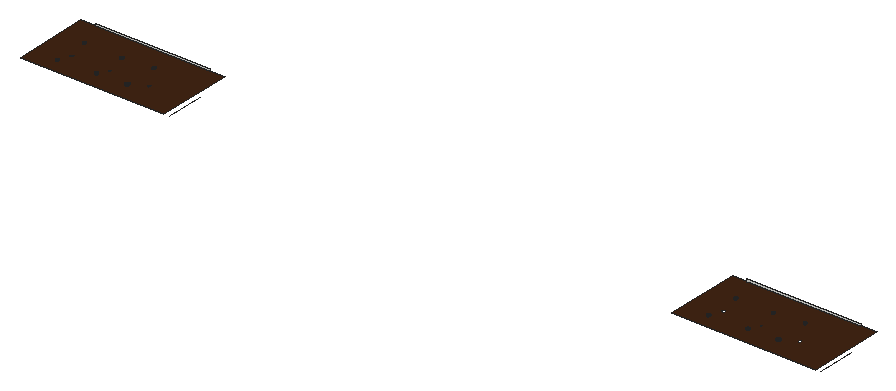
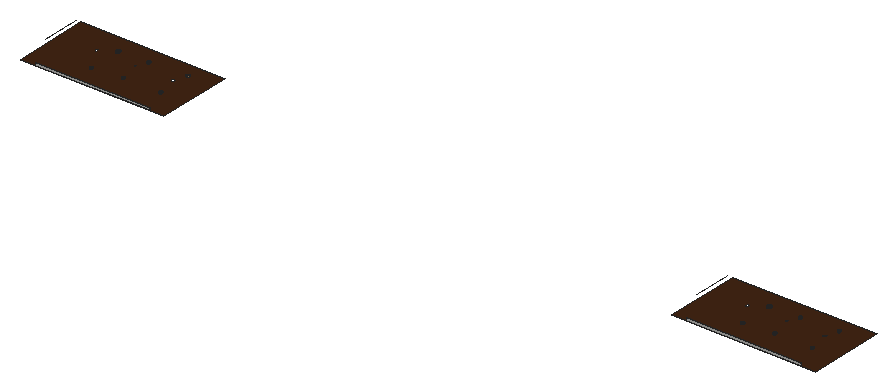
# SketchUp Ruby script. Lengths in inches.
U = 1.inch
M = Sketchup.active_model
def pt(a) = Geom::Point3d.new(a.map { |v| v * U })
def face(e, loops, mat)
  f = e.add_face(loops[0].map { |a| pt(a) })
  loops[1..].each { |l| e.add_face(l.map { |a| pt(a) }).erase! }
  f.material = f.back_material = mat if mat
  f
end
# faces: each face lists its corners as indices into pts; further lists are holes
def faces(e, pts, list, mat = nil) = list.each { |f| face(e, (f[0].is_a?(Array) ? f : [f]).map { |l| l.map { |i| pts[i] } }, mat) }
# xy, xz, yz: faces in a plane at the given z, y or x. An outline is a flat list of corners, or four numbers for a rectangle; further outlines are holes
def ring(l) = l.size == 4 ? [[l[0], l[1]], [l[2], l[1]], [l[2], l[3]], [l[0], l[3]]] : l.each_slice(2).to_a
def flat(e, list, mat, &to3) = list.each { |f| face(e, (f[0].is_a?(Array) ? f : [f]).map { |l| ring(l).map { |u, v| to3.(u, v) } }, mat) }
def xy(e, z, list, mat = nil) = flat(e, list, mat) { |x, y| [x, y, z] }
def xz(e, y, list, mat = nil) = flat(e, list, mat) { |x, z| [x, y, z] }
def yz(e, x, list, mat = nil) = flat(e, list, mat) { |y, z| [x, y, z] }
def lines(e, pts, list) = list.each { |a, b| e.add_line(pt(pts[a]), pt(pts[b])) }
# prism: a flat outline (further loops are holes) pulled along v
def prism(e, loops, v, mat = nil)
  f = face(e, loops, mat); d = Geom::Vector3d.new(v.map { |x| x * U })
  f.pushpull(f.normal.samedirection?(d) ? d.length : -d.length)
end
def box(e, o, s, mat = nil) = prism(e, [[o, [o[0] + s[0], o[1], o[2]], [o[0] + s[0], o[1] + s[1], o[2]], [o[0], o[1] + s[1], o[2]]]], [0, 0, s[2]], mat)
def at(x, y, z, deg = 0) = Geom::Transformation.translation(pt([x, y, z])) * Geom::Transformation.rotation(ORIGIN, Z_AXIS, deg.degrees)
def axes(o, x, y, z) = Geom::Transformation.new([*x, 0, *y, 0, *z, 0, *pt(o).to_a, 1])
def part(name) = M.definitions.add(name)
# library, detail: a bought-in or finely detailed component or shape, given as its bounding box
def library(name, o, s) = part(name).tap { |d| box(d.entities, o, s) }
def detail(e, o, s) = box(e.add_group.entities, o, s)
def put(e, d, t, mat = nil) = e.add_instance(d, t).tap { |i| i.material = mat if mat }
def group(e, t, mat = nil) = e.add_group.tap { |g| g.transformation = t; g.material = mat if mat }.entities
root = M.entities
M.materials.add("[Field Square Tile]").color = [211, 167, 108]
M.materials.add("[Wood Veneer 01]").color = [66, 38, 20]
xy(root,251.5,[[[1990.46,2294.125,2184.6,2396.68],[2030.6,2327.89,2031.39,2328,2032.13,2328.3,2032.76,2328.79,2033.25,2329.43,2033.56,2330.16,2033.66,2330.96,2033.56,2331.75,2033.25,2332.49,2032.76,2333.12,2032.13,2333.61,2031.39,2333.91,2030.6,2334.02,2029.81,2333.91,2029.07,2333.61,2028.43,2333.12,2027.95,2332.49,2027.64,2331.75,2027.54,2330.96,2027.64,2330.16,2027.95,2329.43,2028.43,2328.79,2029.07,2328.3,2029.81,2328],[2134.54,2328.21,2135.25,2328.3,2135.92,2328.57,2136.49,2329.01,2136.92,2329.58,2137.2,2330.24,2137.29,2330.96,2137.2,2331.67,2136.92,2332.33,2136.49,2332.9,2135.92,2333.34,2135.25,2333.61,2134.54,2333.71,2133.83,2333.61,2133.17,2333.34,2132.6,2332.9,2132.16,2332.33,2131.89,2331.67,2131.79,2330.96,2131.89,2330.24,2132.16,2329.58,2132.6,2329.01,2133.17,2328.57,2133.83,2328.3],[2081.97,2328.39,2082.63,2328.48,2083.25,2328.74,2083.78,2329.14,2084.19,2329.68,2084.45,2330.29,2084.53,2330.96,2084.45,2331.62,2084.19,2332.24,2083.78,2332.77,2083.25,2333.18,2082.63,2333.43,2081.97,2333.52,2081.31,2333.43,2080.69,2333.18,2080.16,2332.77,2079.75,2332.24,2079.5,2331.62,2079.41,2330.96,2079.5,2330.29,2079.75,2329.68,2080.16,2329.14,2080.69,2328.74,2081.31,2328.48],[2114.7,2316.65,2115.33,2316.73,2115.92,2316.97,2116.42,2317.36,2116.81,2317.87,2117.05,2318.45,2117.13,2319.08,2117.05,2319.72,2116.81,2320.3,2116.42,2320.81,2115.92,2321.2,2115.33,2321.4375,2114.7,2321.52,2114.07,2321.4375,2113.48,2321.2,2112.97,2320.81,2112.59,2320.3,2112.34,2319.72,2112.26,2319.08,2112.34,2318.45,2112.59,2317.87,2112.97,2317.36,2113.48,2316.97,2114.07,2316.73],[2074.74,2358.2,2075.22,2358.27,2075.67,2358.46,2076.0625,2358.75,2076.36,2359.14,2076.55,2359.59,2076.61,2360.08,2076.55,2360.56,2076.36,2361.02,2076.0625,2361.41,2075.67,2361.7,2075.22,2361.89,2074.74,2361.95,2074.25,2361.89,2073.8,2361.7,2073.41,2361.41,2073.11,2361.02,2072.92,2360.56,2072.86,2360.08,2072.92,2359.59,2073.11,2359.14,2073.41,2358.75,2073.8,2358.46,2074.25,2358.27],[2074.74,2315.39,2075.22,2315.46,2075.67,2315.64,2076.0625,2315.94,2076.36,2316.33,2076.55,2316.78,2076.61,2317.27,2076.55,2317.75,2076.36,2318.2,2076.0625,2318.59,2075.67,2318.89,2075.22,2319.08,2074.74,2319.14,2074.25,2319.08,2073.8,2318.89,2073.41,2318.59,2073.11,2318.2,2072.92,2317.75,2072.86,2317.27,2072.92,2316.78,2073.11,2316.33,2073.41,2315.94,2073.8,2315.64,2074.25,2315.46],[2024.3,2358.2,2024.78,2358.27,2025.24,2358.46,2025.625,2358.75,2025.92,2359.14,2026.11,2359.59,2026.17,2360.08,2026.11,2360.56,2025.92,2361.02,2025.625,2361.41,2025.24,2361.7,2024.78,2361.89,2024.3,2361.95,2023.8125,2361.89,2023.36,2361.7,2022.97,2361.41,2022.67,2361.02,2022.49,2360.56,2022.42,2360.08,2022.49,2359.59,2022.67,2359.14,2022.97,2358.75,2023.36,2358.46,2023.8125,2358.27],[2024.3,2312.27,2024.78,2312.33,2025.24,2312.52,2025.625,2312.82,2025.92,2313.2,2026.11,2313.66,2026.17,2314.14,2026.11,2314.63,2025.92,2315.08,2025.625,2315.47,2025.24,2315.77,2024.78,2315.95,2024.3,2316.02,2023.8125,2315.95,2023.36,2315.77,2022.97,2315.47,2022.67,2315.08,2022.49,2314.63,2022.42,2314.14,2022.49,2313.66,2022.67,2313.2,2022.97,2312.82,2023.36,2312.52,2023.8125,2312.33],[2114.7,2362.38,2115.13,2362.4375,2115.54,2362.6,2115.89,2362.87,2116.16,2363.22,2116.33,2363.63,2116.38,2364.07,2116.33,2364.5,2116.16,2364.91,2115.89,2365.26,2115.54,2365.53,2115.13,2365.7,2114.7,2365.75,2114.26,2365.7,2113.85,2365.53,2113.5,2365.26,2113.24,2364.91,2113.07,2364.5,2113.01,2364.07,2113.07,2363.63,2113.24,2363.22,2113.5,2362.87,2113.85,2362.6,2114.26,2362.4375]],[[2869.21,2294.125,3063.35,2396.68],[2909.35,2327.89,2910.14,2328,2910.88,2328.3,2911.51,2328.79,2912,2329.43,2912.31,2330.16,2912.41,2330.96,2912.31,2331.75,2912,2332.49,2911.51,2333.12,2910.88,2333.61,2910.14,2333.91,2909.35,2334.02,2908.56,2333.91,2907.82,2333.61,2907.18,2333.12,2906.7,2332.49,2906.39,2331.75,2906.29,2330.96,2906.39,2330.16,2906.7,2329.43,2907.18,2328.79,2907.82,2328.3,2908.56,2328],[3013.29,2328.21,3014,2328.3,3014.67,2328.57,3015.24,2329.01,3015.67,2329.58,3015.95,2330.24,3016.04,2330.96,3015.95,2331.67,3015.67,2332.33,3015.24,2332.9,3014.67,2333.34,3014,2333.61,3013.29,2333.71,3012.58,2333.61,3011.92,2333.34,3011.35,2332.9,3010.91,2332.33,3010.64,2331.67,3010.54,2330.96,3010.64,2330.24,3010.91,2329.58,3011.35,2329.01,3011.92,2328.57,3012.58,2328.3],[2960.72,2328.39,2961.38,2328.48,2962,2328.74,2962.53,2329.14,2962.94,2329.68,2963.2,2330.29,2963.28,2330.96,2963.2,2331.62,2962.94,2332.24,2962.53,2332.77,2962,2333.18,2961.38,2333.43,2960.72,2333.52,2960.06,2333.43,2959.44,2333.18,2958.91,2332.77,2958.5,2332.24,2958.25,2331.62,2958.16,2330.96,2958.25,2330.29,2958.5,2329.68,2958.91,2329.14,2959.44,2328.74,2960.06,2328.48],[2993.45,2316.65,2994.08,2316.73,2994.67,2316.97,2995.17,2317.36,2995.56,2317.87,2995.8,2318.45,2995.88,2319.08,2995.8,2319.72,2995.56,2320.3,2995.17,2320.81,2994.67,2321.2,2994.08,2321.4375,2993.45,2321.52,2992.82,2321.4375,2992.23,2321.2,2991.72,2320.81,2991.34,2320.3,2991.09,2319.72,2991.01,2319.08,2991.09,2318.45,2991.34,2317.87,2991.72,2317.36,2992.23,2316.97,2992.82,2316.73],[2903.05,2358.2,2903.53,2358.27,2903.99,2358.46,2904.375,2358.75,2904.67,2359.14,2904.86,2359.59,2904.92,2360.08,2904.86,2360.56,2904.67,2361.02,2904.375,2361.41,2903.99,2361.7,2903.53,2361.89,2903.05,2361.95,2902.5625,2361.89,2902.11,2361.7,2901.72,2361.41,2901.42,2361.02,2901.24,2360.56,2901.17,2360.08,2901.24,2359.59,2901.42,2359.14,2901.72,2358.75,2902.11,2358.46,2902.5625,2358.27],[2953.49,2358.2,2953.97,2358.27,2954.42,2358.46,2954.8125,2358.75,2955.11,2359.14,2955.3,2359.59,2955.36,2360.08,2955.3,2360.56,2955.11,2361.02,2954.8125,2361.41,2954.42,2361.7,2953.97,2361.89,2953.49,2361.95,2953,2361.89,2952.55,2361.7,2952.16,2361.41,2951.86,2361.02,2951.67,2360.56,2951.61,2360.08,2951.67,2359.59,2951.86,2359.14,2952.16,2358.75,2952.55,2358.46,2953,2358.27],[2953.49,2315.39,2953.97,2315.46,2954.42,2315.64,2954.8125,2315.94,2955.11,2316.33,2955.3,2316.78,2955.36,2317.27,2955.3,2317.75,2955.11,2318.2,2954.8125,2318.59,2954.42,2318.89,2953.97,2319.08,2953.49,2319.14,2953,2319.08,2952.55,2318.89,2952.16,2318.59,2951.86,2318.2,2951.67,2317.75,2951.61,2317.27,2951.67,2316.78,2951.86,2316.33,2952.16,2315.94,2952.55,2315.64,2953,2315.46],[2903.05,2312.27,2903.53,2312.33,2903.99,2312.52,2904.375,2312.82,2904.67,2313.2,2904.86,2313.66,2904.92,2314.14,2904.86,2314.63,2904.67,2315.08,2904.375,2315.47,2903.99,2315.77,2903.53,2315.95,2903.05,2316.02,2902.5625,2315.95,2902.11,2315.77,2901.72,2315.47,2901.42,2315.08,2901.24,2314.63,2901.17,2314.14,2901.24,2313.66,2901.42,2313.2,2901.72,2312.82,2902.11,2312.52,2902.5625,2312.33],[2993.45,2362.38,2993.88,2362.4375,2994.29,2362.6,2994.64,2362.87,2994.91,2363.22,2995.08,2363.63,2995.13,2364.07,2995.08,2364.5,2994.91,2364.91,2994.64,2365.26,2994.29,2365.53,2993.88,2365.7,2993.45,2365.75,2993.01,2365.7,2992.6,2365.53,2992.25,2365.26,2991.99,2364.91,2991.82,2364.5,2991.76,2364.07,2991.82,2363.63,2991.99,2363.22,2992.25,2362.87,2992.6,2362.6,2993.01,2362.4375]]],"[Wood Veneer 01]")
xz(root,2396.68,[[2010.28,251.5,2010.34,254.5],[2010.34,251.5,2164.35,254.5],[2889.03,251.5,2889.09,254.5],[2889.09,251.5,3043.1,254.5]])
p = [[2023.8125,2312.33,251.5],[2023.36,2312.52,251.5],[2023.36,2312.52,252.5],[2023.8125,2312.33,252.5],[2024.3,2312.27,251.5],[2024.3,2312.27,252.5],
  [2024.78,2312.33,251.5],[2024.78,2312.33,252.5],[2025.24,2312.52,251.5],[2025.24,2312.52,252.5],[2902.5625,2312.33,251.5],[2902.11,2312.52,251.5],
  [2902.11,2312.52,252.5],[2902.5625,2312.33,252.5],[2903.05,2312.27,251.5],[2903.05,2312.27,252.5],[2903.53,2312.33,251.5],[2903.53,2312.33,252.5],
  [2903.99,2312.52,251.5],[2903.99,2312.52,252.5],[2022.97,2312.82,251.5],[2022.97,2312.82,252.5],[2025.625,2312.82,251.5],[2025.625,2312.82,252.5],
  [2901.72,2312.82,251.5],[2901.72,2312.82,252.5],[2904.375,2312.82,251.5],[2904.375,2312.82,252.5],[2022.67,2313.2,251.5],[2022.67,2313.2,252.5],
  [2025.92,2313.2,251.5],[2025.92,2313.2,252.5],[2901.42,2313.2,251.5],[2901.42,2313.2,252.5],[2904.67,2313.2,251.5],[2904.67,2313.2,252.5],
  [2022.49,2313.66,251.5],[2022.49,2313.66,252.5],[2026.11,2313.66,251.5],[2026.11,2313.66,252.5],[2901.24,2313.66,251.5],[2901.24,2313.66,252.5],
  [2904.86,2313.66,251.5],[2904.86,2313.66,252.5],[2022.42,2314.14,251.5],[2022.42,2314.14,252.5],[2026.17,2314.14,251.5],[2026.17,2314.14,252.5],
  [2901.17,2314.14,251.5],[2901.17,2314.14,252.5],[2904.92,2314.14,251.5],[2904.92,2314.14,252.5],[2022.49,2314.63,251.5],[2022.49,2314.63,252.5],
  [2026.11,2314.63,251.5],[2026.11,2314.63,252.5],[2901.24,2314.63,251.5],[2901.24,2314.63,252.5],[2904.86,2314.63,251.5],[2904.86,2314.63,252.5],
  [2022.67,2315.08,251.5],[2022.67,2315.08,252.5],[2025.92,2315.08,251.5],[2025.92,2315.08,252.5],[2901.42,2315.08,251.5],[2901.42,2315.08,252.5],
  [2904.67,2315.08,251.5],[2904.67,2315.08,252.5],[2022.97,2315.47,251.5],[2022.97,2315.47,252.5],[2025.625,2315.47,251.5],[2025.625,2315.47,252.5],
  [2901.72,2315.47,251.5],[2901.72,2315.47,252.5],[2904.375,2315.47,251.5],[2904.375,2315.47,252.5],[2074.74,2315.39,251.5],[2074.25,2315.46,251.5],
  [2074.25,2315.46,252.5],[2074.74,2315.39,252.5],[2075.22,2315.46,251.5],[2075.22,2315.46,252.5],[2953.49,2315.39,251.5],[2953,2315.46,251.5],
  [2953,2315.46,252.5],[2953.49,2315.39,252.5],[2953.97,2315.46,251.5],[2953.97,2315.46,252.5],[2023.36,2315.77,251.5],[2023.36,2315.77,252.5],
  [2025.24,2315.77,251.5],[2025.24,2315.77,252.5],[2073.8,2315.64,251.5],[2073.8,2315.64,252.5],[2075.67,2315.64,251.5],[2075.67,2315.64,252.5],
  [2902.11,2315.77,251.5],[2902.11,2315.77,252.5],[2903.99,2315.77,251.5],[2903.99,2315.77,252.5],[2952.55,2315.64,251.5],[2952.55,2315.64,252.5],
  [2954.42,2315.64,251.5],[2954.42,2315.64,252.5],[2073.41,2315.94,251.5],[2073.41,2315.94,252.5],[2076.0625,2315.94,251.5],[2076.0625,2315.94,252.5],
  [2952.16,2315.94,251.5],[2952.16,2315.94,252.5],[2954.8125,2315.94,251.5],[2954.8125,2315.94,252.5],[2023.8125,2315.95,251.5],[2023.8125,2315.95,252.5],
  [2024.78,2315.95,251.5],[2024.78,2315.95,252.5],[2902.5625,2315.95,251.5],[2902.5625,2315.95,252.5],[2903.53,2315.95,251.5],[2903.53,2315.95,252.5],
  [2073.11,2316.33,251.5],[2073.11,2316.33,252.5],[2076.36,2316.33,251.5],[2076.36,2316.33,252.5],[2951.86,2316.33,251.5],[2951.86,2316.33,252.5],
  [2955.11,2316.33,251.5],[2955.11,2316.33,252.5],[2024.3,2316.02,251.5],[2024.3,2316.02,252.5],[2903.05,2316.02,251.5],[2903.05,2316.02,252.5],
  [2072.92,2316.78,251.5],[2072.92,2316.78,252.5],[2076.55,2316.78,251.5],[2076.55,2316.78,252.5],[2951.67,2316.78,251.5],[2951.67,2316.78,252.5],
  [2955.3,2316.78,251.5],[2955.3,2316.78,252.5],[2114.7,2316.65,251.5],[2114.07,2316.73,251.5],[2114.07,2316.73,252.5625],[2114.7,2316.65,252.5625],
  [2115.33,2316.73,251.5],[2115.33,2316.73,252.5625],[2993.45,2316.65,251.5],[2992.82,2316.73,251.5],[2992.82,2316.73,252.5625],[2993.45,2316.65,252.5625],
  [2994.08,2316.73,251.5],[2994.08,2316.73,252.5625],[2113.48,2316.97,251.5],[2113.48,2316.97,252.5625],[2115.92,2316.97,251.5],[2115.92,2316.97,252.5625],
  [2992.23,2316.97,251.5],[2992.23,2316.97,252.5625],[2994.67,2316.97,251.5],[2994.67,2316.97,252.5625],[2072.86,2317.27,251.5],[2072.86,2317.27,252.5],
  [2076.61,2317.27,251.5],[2076.61,2317.27,252.5],[2951.61,2317.27,251.5],[2951.61,2317.27,252.5],[2955.36,2317.27,251.5],[2955.36,2317.27,252.5],
  [2112.97,2317.36,251.5],[2112.97,2317.36,252.5625],[2116.42,2317.36,251.5],[2116.42,2317.36,252.5625],[2991.72,2317.36,251.5],[2991.72,2317.36,252.5625],
  [2995.17,2317.36,251.5],[2995.17,2317.36,252.5625],[2072.92,2317.75,251.5],[2072.92,2317.75,252.5],[2076.55,2317.75,251.5],[2076.55,2317.75,252.5],
  [2951.67,2317.75,251.5],[2951.67,2317.75,252.5],[2955.3,2317.75,251.5],[2955.3,2317.75,252.5],[2112.59,2317.87,251.5],[2112.59,2317.87,252.5625],
  [2116.81,2317.87,251.5],[2116.81,2317.87,252.5625],[2991.34,2317.87,251.5],[2991.34,2317.87,252.5625],[2995.56,2317.87,251.5],[2995.56,2317.87,252.5625],
  [2073.11,2318.2,251.5],[2073.11,2318.2,252.5],[2076.36,2318.2,251.5],[2076.36,2318.2,252.5],[2951.86,2318.2,251.5],[2951.86,2318.2,252.5],
  [2955.11,2318.2,251.5],[2955.11,2318.2,252.5],[2112.34,2318.45,251.5],[2112.34,2318.45,252.5625],[2117.05,2318.45,251.5],[2117.05,2318.45,252.5625],
  [2991.09,2318.45,251.5],[2991.09,2318.45,252.5625],[2995.8,2318.45,251.5],[2995.8,2318.45,252.5625],[2073.41,2318.59,251.5],[2073.41,2318.59,252.5],
  [2076.0625,2318.59,251.5],[2076.0625,2318.59,252.5],[2952.16,2318.59,251.5],[2952.16,2318.59,252.5],[2954.8125,2318.59,251.5],[2954.8125,2318.59,252.5],
  [2112.26,2319.08,251.5],[2112.26,2319.08,252.5625],[2117.13,2319.08,251.5],[2117.13,2319.08,252.5625],[2991.01,2319.08,251.5],[2991.01,2319.08,252.5625],
  [2995.88,2319.08,251.5],[2995.88,2319.08,252.5625],[2073.8,2318.89,251.5],[2073.8,2318.89,252.5],[2075.67,2318.89,251.5],[2075.67,2318.89,252.5],
  [2952.55,2318.89,251.5],[2952.55,2318.89,252.5],[2954.42,2318.89,251.5],[2954.42,2318.89,252.5],[2074.25,2319.08,251.5],[2074.25,2319.08,252.5],
  [2075.22,2319.08,251.5],[2075.22,2319.08,252.5],[2953,2319.08,251.5],[2953,2319.08,252.5],[2953.97,2319.08,251.5],[2953.97,2319.08,252.5],
  [2074.74,2319.14,251.5],[2074.74,2319.14,252.5],[2112.34,2319.72,251.5],[2112.34,2319.72,252.5625],[2117.05,2319.72,251.5],[2117.05,2319.72,252.5625],
  [2953.49,2319.14,251.5],[2953.49,2319.14,252.5],[2991.09,2319.72,251.5],[2991.09,2319.72,252.5625],[2995.8,2319.72,251.5],[2995.8,2319.72,252.5625],
  [2112.59,2320.3,251.5],[2112.59,2320.3,252.5625],[2116.81,2320.3,251.5],[2116.81,2320.3,252.5625],[2991.34,2320.3,251.5],[2991.34,2320.3,252.5625],
  [2995.56,2320.3,251.5],[2995.56,2320.3,252.5625],[2112.97,2320.81,251.5],[2112.97,2320.81,252.5625],[2116.42,2320.81,251.5],[2116.42,2320.81,252.5625],
  [2991.72,2320.81,251.5],[2991.72,2320.81,252.5625],[2995.17,2320.81,251.5],[2995.17,2320.81,252.5625],[2113.48,2321.2,251.5],[2113.48,2321.2,252.5625],
  [2115.92,2321.2,251.5],[2115.92,2321.2,252.5625],[2992.23,2321.2,251.5],[2992.23,2321.2,252.5625],[2994.67,2321.2,251.5],[2994.67,2321.2,252.5625],
  [2114.07,2321.4375,251.5],[2114.07,2321.4375,252.5625],[2115.33,2321.4375,251.5],[2115.33,2321.4375,252.5625],[2992.82,2321.4375,251.5],[2992.82,2321.4375,252.5625],
  [2994.08,2321.4375,251.5],[2994.08,2321.4375,252.5625],[2114.7,2321.52,251.5],[2114.7,2321.52,252.5625],[2993.45,2321.52,251.5],[2993.45,2321.52,252.5625],
  [2024.3,2358.2,251.5],[2023.8125,2358.27,251.5],[2023.8125,2358.27,252.5],[2024.3,2358.2,252.5],[2024.78,2358.27,251.5],[2024.78,2358.27,252.5],
  [2074.74,2358.2,251.5],[2074.25,2358.27,251.5],[2074.25,2358.27,252.5],[2074.74,2358.2,252.5],[2075.22,2358.27,251.5],[2075.22,2358.27,252.5],
  [2903.05,2358.2,251.5],[2902.5625,2358.27,251.5],[2902.5625,2358.27,252.5],[2903.05,2358.2,252.5],[2903.53,2358.27,251.5],[2903.53,2358.27,252.5],
  [2953.49,2358.2,251.5],[2953,2358.27,251.5],[2953,2358.27,252.5],[2953.49,2358.2,252.5],[2953.97,2358.27,251.5],[2953.97,2358.27,252.5],
  [2023.36,2358.46,251.5],[2023.36,2358.46,252.5],[2025.24,2358.46,251.5],[2025.24,2358.46,252.5],[2073.8,2358.46,251.5],[2073.8,2358.46,252.5],
  [2075.67,2358.46,251.5],[2075.67,2358.46,252.5],[2902.11,2358.46,251.5],[2902.11,2358.46,252.5],[2903.99,2358.46,251.5],[2903.99,2358.46,252.5],
  [2952.55,2358.46,251.5],[2952.55,2358.46,252.5],[2954.42,2358.46,251.5],[2954.42,2358.46,252.5],[2022.97,2358.75,251.5],[2022.97,2358.75,252.5],
  [2025.625,2358.75,251.5],[2025.625,2358.75,252.5],[2073.41,2358.75,251.5],[2073.41,2358.75,252.5],[2076.0625,2358.75,251.5],[2076.0625,2358.75,252.5],
  [2901.72,2358.75,251.5],[2901.72,2358.75,252.5],[2904.375,2358.75,251.5],[2904.375,2358.75,252.5],[2952.16,2358.75,251.5],[2952.16,2358.75,252.5],
  [2954.8125,2358.75,251.5],[2954.8125,2358.75,252.5],[2022.67,2359.14,251.5],[2022.67,2359.14,252.5],[2025.92,2359.14,251.5],[2025.92,2359.14,252.5],
  [2073.11,2359.14,251.5],[2073.11,2359.14,252.5],[2076.36,2359.14,251.5],[2076.36,2359.14,252.5],[2901.42,2359.14,251.5],[2901.42,2359.14,252.5],
  [2904.67,2359.14,251.5],[2904.67,2359.14,252.5],[2951.86,2359.14,251.5],[2951.86,2359.14,252.5],[2955.11,2359.14,251.5],[2955.11,2359.14,252.5],
  [2022.49,2359.59,251.5],[2022.49,2359.59,252.5],[2026.11,2359.59,251.5],[2026.11,2359.59,252.5],[2072.92,2359.59,251.5],[2072.92,2359.59,252.5],
  [2076.55,2359.59,251.5],[2076.55,2359.59,252.5],[2901.24,2359.59,251.5],[2901.24,2359.59,252.5],[2904.86,2359.59,251.5],[2904.86,2359.59,252.5],
  [2951.67,2359.59,251.5],[2951.67,2359.59,252.5],[2955.3,2359.59,251.5],[2955.3,2359.59,252.5],[2022.42,2360.08,251.5],[2022.42,2360.08,252.5],
  [2026.17,2360.08,251.5],[2026.17,2360.08,252.5],[2072.86,2360.08,251.5],[2072.86,2360.08,252.5],[2076.61,2360.08,251.5],[2076.61,2360.08,252.5],
  [2901.17,2360.08,251.5],[2901.17,2360.08,252.5],[2904.92,2360.08,251.5],[2904.92,2360.08,252.5],[2951.61,2360.08,251.5],[2951.61,2360.08,252.5],
  [2955.36,2360.08,251.5],[2955.36,2360.08,252.5],[2022.49,2360.56,251.5],[2022.49,2360.56,252.5],[2026.11,2360.56,251.5],[2026.11,2360.56,252.5],
  [2072.92,2360.56,251.5],[2072.92,2360.56,252.5],[2076.55,2360.56,251.5],[2076.55,2360.56,252.5],[2901.24,2360.56,251.5],[2901.24,2360.56,252.5],
  [2904.86,2360.56,251.5],[2904.86,2360.56,252.5],[2951.67,2360.56,251.5],[2951.67,2360.56,252.5],[2955.3,2360.56,251.5],[2955.3,2360.56,252.5],
  [2022.67,2361.02,251.5],[2022.67,2361.02,252.5],[2025.92,2361.02,251.5],[2025.92,2361.02,252.5],[2073.11,2361.02,251.5],[2073.11,2361.02,252.5],
  [2076.36,2361.02,251.5],[2076.36,2361.02,252.5],[2901.42,2361.02,251.5],[2901.42,2361.02,252.5],[2904.67,2361.02,251.5],[2904.67,2361.02,252.5],
  [2951.86,2361.02,251.5],[2951.86,2361.02,252.5],[2955.11,2361.02,251.5],[2955.11,2361.02,252.5],[2022.97,2361.41,251.5],[2022.97,2361.41,252.5],
  [2025.625,2361.41,251.5],[2025.625,2361.41,252.5],[2073.41,2361.41,251.5],[2073.41,2361.41,252.5],[2076.0625,2361.41,251.5],[2076.0625,2361.41,252.5],
  [2901.72,2361.41,251.5],[2901.72,2361.41,252.5],[2904.375,2361.41,251.5],[2904.375,2361.41,252.5],[2952.16,2361.41,251.5],[2952.16,2361.41,252.5],
  [2954.8125,2361.41,251.5],[2954.8125,2361.41,252.5],[2023.36,2361.7,251.5],[2023.36,2361.7,252.5],[2025.24,2361.7,251.5],[2025.24,2361.7,252.5],
  [2073.8,2361.7,251.5],[2073.8,2361.7,252.5],[2075.67,2361.7,251.5],[2075.67,2361.7,252.5],[2902.11,2361.7,251.5],[2902.11,2361.7,252.5],
  [2903.99,2361.7,251.5],[2903.99,2361.7,252.5],[2952.55,2361.7,251.5],[2952.55,2361.7,252.5],[2954.42,2361.7,251.5],[2954.42,2361.7,252.5],
  [2023.8125,2361.89,251.5],[2023.8125,2361.89,252.5],[2024.78,2361.89,251.5],[2024.78,2361.89,252.5],[2074.25,2361.89,251.5],[2074.25,2361.89,252.5],
  [2075.22,2361.89,251.5],[2075.22,2361.89,252.5],[2902.5625,2361.89,251.5],[2902.5625,2361.89,252.5],[2903.53,2361.89,251.5],[2903.53,2361.89,252.5],
  [2953,2361.89,251.5],[2953,2361.89,252.5],[2953.97,2361.89,251.5],[2953.97,2361.89,252.5],[2024.3,2361.95,251.5],[2024.3,2361.95,252.5],
  [2074.74,2361.95,251.5],[2074.74,2361.95,252.5],[2903.05,2361.95,251.5],[2903.05,2361.95,252.5],[2953.49,2361.95,251.5],[2953.49,2361.95,252.5],
  [2114.26,2362.4375,251.5],[2113.85,2362.6,251.5],[2113.85,2362.6,252.4375],[2114.26,2362.4375,252.4375],[2114.7,2362.38,251.5],[2114.7,2362.38,252.4375],
  [2115.13,2362.4375,251.5],[2115.13,2362.4375,252.4375],[2115.54,2362.6,251.5],[2115.54,2362.6,252.4375],[2993.01,2362.4375,251.5],[2992.6,2362.6,251.5],
  [2992.6,2362.6,252.4375],[2993.01,2362.4375,252.4375],[2993.45,2362.38,251.5],[2993.45,2362.38,252.4375],[2993.88,2362.4375,251.5],[2993.88,2362.4375,252.4375],
  [2994.29,2362.6,251.5],[2994.29,2362.6,252.4375],[2113.5,2362.87,251.5],[2113.5,2362.87,252.4375],[2115.89,2362.87,251.5],[2115.89,2362.87,252.4375],
  [2992.25,2362.87,251.5],[2992.25,2362.87,252.4375],[2994.64,2362.87,251.5],[2994.64,2362.87,252.4375],[2113.24,2363.22,251.5],[2113.24,2363.22,252.4375],
  [2116.16,2363.22,251.5],[2116.16,2363.22,252.4375],[2991.99,2363.22,251.5],[2991.99,2363.22,252.4375],[2994.91,2363.22,251.5],[2994.91,2363.22,252.4375],
  [2113.07,2363.63,251.5],[2113.07,2363.63,252.4375],[2116.33,2363.63,251.5],[2116.33,2363.63,252.4375],[2991.82,2363.63,251.5],[2991.82,2363.63,252.4375],
  [2995.08,2363.63,251.5],[2995.08,2363.63,252.4375],[2113.01,2364.07,251.5],[2113.01,2364.07,252.4375],[2116.38,2364.07,251.5],[2116.38,2364.07,252.4375],
  [2991.76,2364.07,251.5],[2991.76,2364.07,252.4375],[2995.13,2364.07,251.5],[2995.13,2364.07,252.4375],[2113.07,2364.5,251.5],[2113.07,2364.5,252.4375],
  [2116.33,2364.5,251.5],[2116.33,2364.5,252.4375],[2991.82,2364.5,251.5],[2991.82,2364.5,252.4375],[2995.08,2364.5,251.5],[2995.08,2364.5,252.4375],
  [2113.24,2364.91,251.5],[2113.24,2364.91,252.4375],[2116.16,2364.91,251.5],[2116.16,2364.91,252.4375],[2991.99,2364.91,251.5],[2991.99,2364.91,252.4375],
  [2994.91,2364.91,251.5],[2994.91,2364.91,252.4375],[2113.5,2365.26,251.5],[2113.5,2365.26,252.4375],[2115.89,2365.26,251.5],[2115.89,2365.26,252.4375],
  [2992.25,2365.26,251.5],[2992.25,2365.26,252.4375],[2994.64,2365.26,251.5],[2994.64,2365.26,252.4375],[2113.85,2365.53,251.5],[2113.85,2365.53,252.4375],
  [2115.54,2365.53,251.5],[2115.54,2365.53,252.4375],[2992.6,2365.53,251.5],[2992.6,2365.53,252.4375],[2994.29,2365.53,251.5],[2994.29,2365.53,252.4375],
  [2114.26,2365.7,251.5],[2114.26,2365.7,252.4375],[2115.13,2365.7,251.5],[2115.13,2365.7,252.4375],[2993.01,2365.7,251.5],[2993.01,2365.7,252.4375],
  [2993.88,2365.7,251.5],[2993.88,2365.7,252.4375],[2114.7,2365.75,251.5],[2114.7,2365.75,252.4375],[2993.45,2365.75,251.5],[2993.45,2365.75,252.4375],
  [2191.47,2346.71,251.5],[2191.47,2294.125,251.5],[3070.22,2346.71,251.5],[3070.22,2294.125,251.5]]
faces(root,p,[[0,1,2,3],[4,0,3,5],[6,4,5,7],[8,6,7,9],[10,11,12,13],[14,10,13,15],[16,14,15,17],[18,16,17,19],
  [1,20,21,2],[22,8,9,23],[11,24,25,12],[26,18,19,27],[20,28,29,21],[30,22,23,31],[24,32,33,25],[34,26,27,35],
  [28,36,37,29],[38,30,31,39],[32,40,41,33],[42,34,35,43],[36,44,45,37],[46,38,39,47],[40,48,49,41],[50,42,43,51],
  [44,52,53,45],[54,46,47,55],[48,56,57,49],[58,50,51,59],[52,60,61,53],[62,54,55,63],[56,64,65,57],[66,58,59,67],
  [60,68,69,61],[70,62,63,71],[64,72,73,65],[74,66,67,75],[76,77,78,79],[80,76,79,81],[82,83,84,85],[86,82,85,87],
  [68,88,89,69],[90,70,71,91],[77,92,93,78],[94,80,81,95],[72,96,97,73],[98,74,75,99],[83,100,101,84],[102,86,87,103],
  [92,104,105,93],[106,94,95,107],[100,108,109,101],[110,102,103,111],[88,112,113,89],[114,90,91,115],[96,116,117,97],[118,98,99,119],
  [104,120,121,105],[122,106,107,123],[108,124,125,109],[126,110,111,127],[112,128,129,113],[128,114,115,129],[116,130,131,117],[130,118,119,131],
  [120,132,133,121],[134,122,123,135],[124,136,137,125],[138,126,127,139],[140,141,142,143],[144,140,143,145],[146,147,148,149],[150,146,149,151],
  [141,152,153,142],[154,144,145,155],[147,156,157,148],[158,150,151,159],[132,160,161,133],[162,134,135,163],[136,164,165,137],[166,138,139,167],
  [152,168,169,153],[170,154,155,171],[156,172,173,157],[174,158,159,175],[160,176,177,161],[178,162,163,179],[164,180,181,165],[182,166,167,183],
  [168,184,185,169],[186,170,171,187],[172,188,189,173],[190,174,175,191],[176,192,193,177],[194,178,179,195],[180,196,197,181],[198,182,183,199],
  [184,200,201,185],[202,186,187,203],[188,204,205,189],[206,190,191,207],[192,208,209,193],[210,194,195,211],[196,212,213,197],[214,198,199,215],
  [200,216,217,201],[218,202,203,219],[204,220,221,205],[222,206,207,223],[208,224,225,209],[226,210,211,227],[212,228,229,213],[230,214,215,231],
  [224,232,233,225],[234,226,227,235],[228,236,237,229],[238,230,231,239],[232,240,241,233],[240,234,235,241],[216,242,243,217],[244,218,219,245],
  [236,246,247,237],[246,238,239,247],[220,248,249,221],[250,222,223,251],[242,252,253,243],[254,244,245,255],[248,256,257,249],[258,250,251,259],
  [252,260,261,253],[262,254,255,263],[256,264,265,257],[266,258,259,267],[260,268,269,261],[270,262,263,271],[264,272,273,265],[274,266,267,275],
  [268,276,277,269],[278,270,271,279],[272,280,281,273],[282,274,275,283],[276,284,285,277],[284,278,279,285],[280,286,287,281],[286,282,283,287],
  [288,289,290,291],[292,288,291,293],[294,295,296,297],[298,294,297,299],[300,301,302,303],[304,300,303,305],[306,307,308,309],[310,306,309,311],
  [289,312,313,290],[314,292,293,315],[295,316,317,296],[318,298,299,319],[301,320,321,302],[322,304,305,323],[307,324,325,308],[326,310,311,327],
  [312,328,329,313],[330,314,315,331],[316,332,333,317],[334,318,319,335],[320,336,337,321],[338,322,323,339],[324,340,341,325],[342,326,327,343],
  [328,344,345,329],[346,330,331,347],[332,348,349,333],[350,334,335,351],[336,352,353,337],[354,338,339,355],[340,356,357,341],[358,342,343,359],
  [344,360,361,345],[362,346,347,363],[348,364,365,349],[366,350,351,367],[352,368,369,353],[370,354,355,371],[356,372,373,357],[374,358,359,375],
  [360,376,377,361],[378,362,363,379],[364,380,381,365],[382,366,367,383],[368,384,385,369],[386,370,371,387],[372,388,389,373],[390,374,375,391],
  [376,392,393,377],[394,378,379,395],[380,396,397,381],[398,382,383,399],[384,400,401,385],[402,386,387,403],[388,404,405,389],[406,390,391,407],
  [392,408,409,393],[410,394,395,411],[396,412,413,397],[414,398,399,415],[400,416,417,401],[418,402,403,419],[404,420,421,405],[422,406,407,423],
  [408,424,425,409],[426,410,411,427],[412,428,429,413],[430,414,415,431],[416,432,433,417],[434,418,419,435],[420,436,437,421],[438,422,423,439],
  [424,440,441,425],[442,426,427,443],[428,444,445,429],[446,430,431,447],[432,448,449,433],[450,434,435,451],[436,452,453,437],[454,438,439,455],
  [440,456,457,441],[458,442,443,459],[444,460,461,445],[462,446,447,463],[448,464,465,449],[466,450,451,467],[452,468,469,453],[470,454,455,471],
  [456,472,473,457],[472,458,459,473],[460,474,475,461],[474,462,463,475],[464,476,477,465],[476,466,467,477],[468,478,479,469],[478,470,471,479],
  [480,481,482,483],[484,480,483,485],[486,484,485,487],[488,486,487,489],[490,491,492,493],[494,490,493,495],[496,494,495,497],[498,496,497,499],
  [481,500,501,482],[502,488,489,503],[491,504,505,492],[506,498,499,507],[500,508,509,501],[510,502,503,511],[504,512,513,505],[514,506,507,515],
  [508,516,517,509],[518,510,511,519],[512,520,521,513],[522,514,515,523],[516,524,525,517],[526,518,519,527],[520,528,529,521],[530,522,523,531],
  [524,532,533,525],[534,526,527,535],[528,536,537,529],[538,530,531,539],[532,540,541,533],[542,534,535,543],[536,544,545,537],[546,538,539,547],
  [540,548,549,541],[550,542,543,551],[544,552,553,545],[554,546,547,555],[548,556,557,549],[558,550,551,559],[552,560,561,553],[562,554,555,563],
  [556,564,565,557],[566,558,559,567],[560,568,569,561],[570,562,563,571],[564,572,573,565],[572,566,567,573],[568,574,575,569],[574,570,571,575]],"[Field Square Tile]")
lines(root,p,[[576,577],[578,579]])
